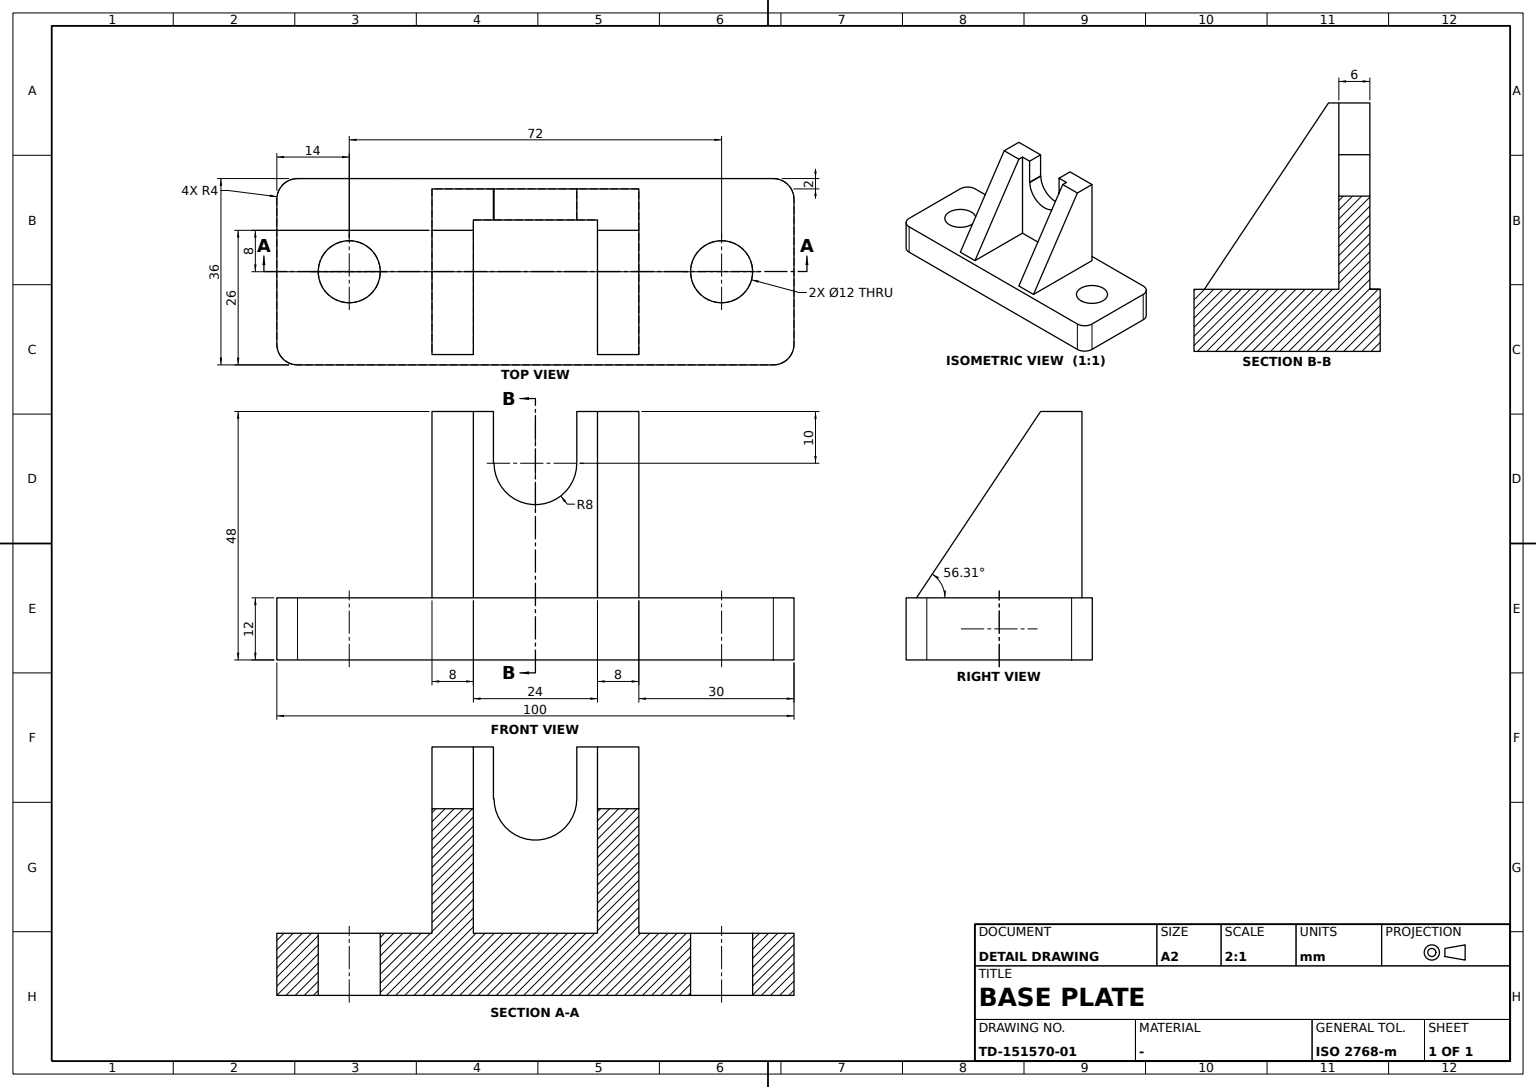
ISO-10303-21;
HEADER;
FILE_DESCRIPTION((''),'2;1');
FILE_NAME('','',(''),(''),'','','');
FILE_SCHEMA(('AUTOMOTIVE_DESIGN'));
ENDSEC;
DATA;
#1=APPLICATION_CONTEXT('');
#2=PRODUCT_CONTEXT('',#1,'mechanical');
#3=PRODUCT('','','',(#2));
#4=PRODUCT_DEFINITION_FORMATION('','',#3);
#5=PRODUCT_DEFINITION_CONTEXT('',#1,'design');
#6=PRODUCT_DEFINITION('','',#4,#5);
#7=PRODUCT_DEFINITION_SHAPE('','',#6);
#8=(LENGTH_UNIT()NAMED_UNIT(*)SI_UNIT(.MILLI.,.METRE.));
#9=(NAMED_UNIT(*)PLANE_ANGLE_UNIT()SI_UNIT($,.RADIAN.));
#10=(NAMED_UNIT(*)SI_UNIT($,.STERADIAN.)SOLID_ANGLE_UNIT());
#11=UNCERTAINTY_MEASURE_WITH_UNIT(LENGTH_MEASURE(0.005),#8,'distance_accuracy_value','');
#12=(GEOMETRIC_REPRESENTATION_CONTEXT(3)GLOBAL_UNCERTAINTY_ASSIGNED_CONTEXT((#11))GLOBAL_UNIT_ASSIGNED_CONTEXT((#8,#9,#10))REPRESENTATION_CONTEXT('',''));
#13=CARTESIAN_POINT('',(32.,100.,12.));
#14=VERTEX_POINT('',#13);
#15=CARTESIAN_POINT('',(4.,100.,12.));
#16=VERTEX_POINT('',#15);
#17=CARTESIAN_POINT('',(0.,100.,12.));
#18=DIRECTION('',(-1.,0.,0.));
#19=VECTOR('',#18,1000.);
#20=LINE('',#17,#19);
#21=EDGE_CURVE('',#14,#16,#20,.T.);
#22=ORIENTED_EDGE('',*,*,#21,.F.);
#23=CARTESIAN_POINT('',(32.,100.,0.));
#24=VERTEX_POINT('',#23);
#25=CARTESIAN_POINT('',(32.,100.,6.));
#26=DIRECTION('',(0.,0.,1.));
#27=VECTOR('',#26,1000.);
#28=LINE('',#25,#27);
#29=EDGE_CURVE('',#24,#14,#28,.T.);
#30=ORIENTED_EDGE('',*,*,#29,.F.);
#31=CARTESIAN_POINT('',(4.,100.,0.));
#32=VERTEX_POINT('',#31);
#33=CARTESIAN_POINT('',(0.,100.,0.));
#34=LINE('',#33,#19);
#35=EDGE_CURVE('',#24,#32,#34,.T.);
#36=ORIENTED_EDGE('',*,*,#35,.T.);
#37=CARTESIAN_POINT('',(4.,100.,6.));
#38=LINE('',#37,#27);
#39=EDGE_CURVE('',#32,#16,#38,.T.);
#40=ORIENTED_EDGE('',*,*,#39,.T.);
#41=EDGE_LOOP('',(#22,#30,#36,#40));
#42=FACE_BOUND('',#41,.T.);
#43=CARTESIAN_POINT('',(36.,100.,0.));
#44=DIRECTION('',(0.,1.,0.));
#45=AXIS2_PLACEMENT_3D('',#43,#44,#18);
#46=PLANE('',#45);
#47=ADVANCED_FACE('',(#42),#46,.T.);
#48=CARTESIAN_POINT('',(2.,70.,12.));
#49=VERTEX_POINT('',#48);
#50=CARTESIAN_POINT('',(2.,70.,48.));
#51=VERTEX_POINT('',#50);
#52=LINE('',#48,#27);
#53=EDGE_CURVE('',#49,#51,#52,.T.);
#54=ORIENTED_EDGE('',*,*,#53,.T.);
#55=CARTESIAN_POINT('',(10.,70.,48.));
#56=VERTEX_POINT('',#55);
#57=DIRECTION('',(1.,0.,0.));
#58=VECTOR('',#57,1000.);
#59=LINE('',#50,#58);
#60=EDGE_CURVE('',#51,#56,#59,.T.);
#61=ORIENTED_EDGE('',*,*,#60,.T.);
#62=CARTESIAN_POINT('',(34.,70.,12.));
#63=VERTEX_POINT('',#62);
#64=CARTESIAN_POINT('',(29.076923,70.,19.384615));
#65=DIRECTION('',(-0.554700196,0.,0.832050294));
#66=VECTOR('',#65,1000.);
#67=LINE('',#64,#66);
#68=EDGE_CURVE('',#63,#56,#67,.T.);
#69=ORIENTED_EDGE('',*,*,#68,.F.);
#70=CARTESIAN_POINT('',(0.,70.,12.));
#71=LINE('',#70,#19);
#72=EDGE_CURVE('',#63,#49,#71,.T.);
#73=ORIENTED_EDGE('',*,*,#72,.T.);
#74=EDGE_LOOP('',(#54,#61,#69,#73));
#75=FACE_BOUND('',#74,.T.);
#76=CARTESIAN_POINT('',(0.,70.,0.));
#77=AXIS2_PLACEMENT_3D('',#76,#44,#18);
#78=PLANE('',#77);
#79=ADVANCED_FACE('',(#75),#78,.T.);
#80=CARTESIAN_POINT('',(36.,96.,12.));
#81=VERTEX_POINT('',#80);
#82=CARTESIAN_POINT('',(32.,96.,12.));
#83=AXIS2_PLACEMENT_3D('',#82,#26,#57);
#84=CIRCLE('',#83,4.);
#85=EDGE_CURVE('',#81,#14,#84,.T.);
#86=ORIENTED_EDGE('',*,*,#85,.F.);
#87=CARTESIAN_POINT('',(36.,96.,0.));
#88=VERTEX_POINT('',#87);
#89=CARTESIAN_POINT('',(36.,96.,6.));
#90=LINE('',#89,#27);
#91=EDGE_CURVE('',#88,#81,#90,.T.);
#92=ORIENTED_EDGE('',*,*,#91,.F.);
#93=CARTESIAN_POINT('',(32.,96.,0.));
#94=AXIS2_PLACEMENT_3D('',#93,#26,#57);
#95=CIRCLE('',#94,4.);
#96=EDGE_CURVE('',#88,#24,#95,.T.);
#97=ORIENTED_EDGE('',*,*,#96,.T.);
#98=ORIENTED_EDGE('',*,*,#29,.T.);
#99=EDGE_LOOP('',(#86,#92,#97,#98));
#100=FACE_BOUND('',#99,.T.);
#101=CARTESIAN_POINT('',(32.,96.,6.));
#102=AXIS2_PLACEMENT_3D('',#101,#26,#44);
#103=CYLINDRICAL_SURFACE('',#102,4.);
#104=ADVANCED_FACE('',(#100),#103,.T.);
#105=CARTESIAN_POINT('',(0.,4.,12.));
#106=VERTEX_POINT('',#105);
#107=CARTESIAN_POINT('',(0.,96.,12.));
#108=VERTEX_POINT('',#107);
#109=CARTESIAN_POINT('',(0.,0.,12.));
#110=VECTOR('',#44,1000.);
#111=LINE('',#109,#110);
#112=EDGE_CURVE('',#106,#108,#111,.T.);
#113=ORIENTED_EDGE('',*,*,#112,.T.);
#114=CARTESIAN_POINT('',(0.,96.,0.));
#115=VERTEX_POINT('',#114);
#116=CARTESIAN_POINT('',(0.,96.,6.));
#117=LINE('',#116,#27);
#118=EDGE_CURVE('',#115,#108,#117,.T.);
#119=ORIENTED_EDGE('',*,*,#118,.F.);
#120=CARTESIAN_POINT('',(0.,4.,0.));
#121=VERTEX_POINT('',#120);
#122=CARTESIAN_POINT('',(0.,0.,0.));
#123=LINE('',#122,#110);
#124=EDGE_CURVE('',#121,#115,#123,.T.);
#125=ORIENTED_EDGE('',*,*,#124,.F.);
#126=CARTESIAN_POINT('',(0.,4.,6.));
#127=LINE('',#126,#27);
#128=EDGE_CURVE('',#121,#106,#127,.T.);
#129=ORIENTED_EDGE('',*,*,#128,.T.);
#130=EDGE_LOOP('',(#113,#119,#125,#129));
#131=FACE_BOUND('',#130,.T.);
#132=AXIS2_PLACEMENT_3D('',#122,#57,#44);
#133=PLANE('',#132);
#134=ADVANCED_FACE('',(#131),#133,.F.);
#135=CARTESIAN_POINT('',(2.,58.,48.));
#136=VERTEX_POINT('',#135);
#137=CARTESIAN_POINT('',(2.,58.,38.));
#138=VERTEX_POINT('',#137);
#139=CARTESIAN_POINT('',(2.,58.,12.));
#140=DIRECTION('',(0.,0.,-1.));
#141=VECTOR('',#140,1000.);
#142=LINE('',#139,#141);
#143=EDGE_CURVE('',#136,#138,#142,.T.);
#144=ORIENTED_EDGE('',*,*,#143,.T.);
#145=CARTESIAN_POINT('',(8.,58.,38.));
#146=VERTEX_POINT('',#145);
#147=CARTESIAN_POINT('',(19.66,58.,38.));
#148=LINE('',#147,#19);
#149=EDGE_CURVE('',#138,#146,#148,.F.);
#150=ORIENTED_EDGE('',*,*,#149,.T.);
#151=CARTESIAN_POINT('',(8.,58.,48.));
#152=VERTEX_POINT('',#151);
#153=CARTESIAN_POINT('',(8.,58.,48.236969));
#154=LINE('',#153,#27);
#155=EDGE_CURVE('',#146,#152,#154,.T.);
#156=ORIENTED_EDGE('',*,*,#155,.T.);
#157=LINE('',#135,#58);
#158=EDGE_CURVE('',#136,#152,#157,.T.);
#159=ORIENTED_EDGE('',*,*,#158,.F.);
#160=EDGE_LOOP('',(#144,#150,#156,#159));
#161=FACE_BOUND('',#160,.T.);
#162=CARTESIAN_POINT('',(2.,58.,48.236969));
#163=DIRECTION('',(0.,-1.,0.));
#164=AXIS2_PLACEMENT_3D('',#162,#163,#140);
#165=PLANE('',#164);
#166=ADVANCED_FACE('',(#161),#165,.T.);
#167=CARTESIAN_POINT('',(2.,41.879669,48.));
#168=VERTEX_POINT('',#167);
#169=CARTESIAN_POINT('',(8.,41.879669,48.));
#170=VERTEX_POINT('',#169);
#171=LINE('',#167,#58);
#172=EDGE_CURVE('',#168,#170,#171,.T.);
#173=ORIENTED_EDGE('',*,*,#172,.T.);
#174=CARTESIAN_POINT('',(8.,41.879669,38.));
#175=VERTEX_POINT('',#174);
#176=LINE('',#169,#27);
#177=EDGE_CURVE('',#175,#170,#176,.T.);
#178=ORIENTED_EDGE('',*,*,#177,.F.);
#179=CARTESIAN_POINT('',(2.,41.879669,38.));
#180=VERTEX_POINT('',#179);
#181=LINE('',#179,#58);
#182=EDGE_CURVE('',#180,#175,#181,.T.);
#183=ORIENTED_EDGE('',*,*,#182,.F.);
#184=CARTESIAN_POINT('',(2.,41.879669,12.));
#185=LINE('',#184,#27);
#186=EDGE_CURVE('',#180,#168,#185,.T.);
#187=ORIENTED_EDGE('',*,*,#186,.T.);
#188=EDGE_LOOP('',(#173,#178,#183,#187));
#189=FACE_BOUND('',#188,.T.);
#190=AXIS2_PLACEMENT_3D('',#179,#44,#26);
#191=PLANE('',#190);
#192=ADVANCED_FACE('',(#189),#191,.T.);
#193=CARTESIAN_POINT('',(8.,62.,48.));
#194=VERTEX_POINT('',#193);
#195=CARTESIAN_POINT('',(8.,62.,12.));
#196=VERTEX_POINT('',#195);
#197=LINE('',#193,#141);
#198=EDGE_CURVE('',#194,#196,#197,.T.);
#199=ORIENTED_EDGE('',*,*,#198,.T.);
#200=CARTESIAN_POINT('',(34.,62.,12.));
#201=VERTEX_POINT('',#200);
#202=LINE('',#195,#58);
#203=EDGE_CURVE('',#196,#201,#202,.T.);
#204=ORIENTED_EDGE('',*,*,#203,.T.);
#205=CARTESIAN_POINT('',(10.,62.,48.));
#206=VERTEX_POINT('',#205);
#207=CARTESIAN_POINT('',(9.384615,62.,48.923077));
#208=LINE('',#207,#66);
#209=EDGE_CURVE('',#201,#206,#208,.T.);
#210=ORIENTED_EDGE('',*,*,#209,.T.);
#211=CARTESIAN_POINT('',(2.,62.,48.));
#212=LINE('',#211,#58);
#213=EDGE_CURVE('',#194,#206,#212,.T.);
#214=ORIENTED_EDGE('',*,*,#213,.F.);
#215=EDGE_LOOP('',(#199,#204,#210,#214));
#216=FACE_BOUND('',#215,.T.);
#217=AXIS2_PLACEMENT_3D('',#193,#44,#57);
#218=PLANE('',#217);
#219=ADVANCED_FACE('',(#216),#218,.F.);
#220=ORIENTED_EDGE('',*,*,#68,.T.);
#221=CARTESIAN_POINT('',(10.,100.,48.));
#222=VECTOR('',#163,1000.);
#223=LINE('',#221,#222);
#224=EDGE_CURVE('',#56,#206,#223,.T.);
#225=ORIENTED_EDGE('',*,*,#224,.T.);
#226=ORIENTED_EDGE('',*,*,#209,.F.);
#227=CARTESIAN_POINT('',(34.,0.,12.));
#228=LINE('',#227,#222);
#229=EDGE_CURVE('',#63,#201,#228,.T.);
#230=ORIENTED_EDGE('',*,*,#229,.F.);
#231=EDGE_LOOP('',(#220,#225,#226,#230));
#232=FACE_BOUND('',#231,.T.);
#233=DIRECTION('',(-0.832050294,0.,-0.554700196));
#234=DIRECTION('',(0.554700196,0.,-0.832050294));
#235=AXIS2_PLACEMENT_3D('',#221,#233,#234);
#236=PLANE('',#235);
#237=ADVANCED_FACE('',(#232),#236,.F.);
#238=CARTESIAN_POINT('',(2.,42.,38.));
#239=VERTEX_POINT('',#238);
#240=CARTESIAN_POINT('',(2.,50.,38.));
#241=AXIS2_PLACEMENT_3D('',#240,#57,#140);
#242=CIRCLE('',#241,8.);
#243=EDGE_CURVE('',#138,#239,#242,.F.);
#244=ORIENTED_EDGE('',*,*,#243,.T.);
#245=CARTESIAN_POINT('',(8.,42.,38.));
#246=VERTEX_POINT('',#245);
#247=LINE('',#238,#19);
#248=EDGE_CURVE('',#239,#246,#247,.F.);
#249=ORIENTED_EDGE('',*,*,#248,.T.);
#250=CARTESIAN_POINT('',(8.,50.,38.));
#251=AXIS2_PLACEMENT_3D('',#250,#57,#140);
#252=CIRCLE('',#251,8.);
#253=EDGE_CURVE('',#246,#146,#252,.T.);
#254=ORIENTED_EDGE('',*,*,#253,.T.);
#255=ORIENTED_EDGE('',*,*,#149,.F.);
#256=EDGE_LOOP('',(#244,#249,#254,#255));
#257=FACE_BOUND('',#256,.T.);
#258=CARTESIAN_POINT('',(19.66,50.,38.));
#259=AXIS2_PLACEMENT_3D('',#258,#18,#163);
#260=CYLINDRICAL_SURFACE('',#259,8.);
#261=ADVANCED_FACE('',(#257),#260,.F.);
#262=CARTESIAN_POINT('',(36.,4.,0.));
#263=VERTEX_POINT('',#262);
#264=CARTESIAN_POINT('',(36.,4.,12.));
#265=VERTEX_POINT('',#264);
#266=CARTESIAN_POINT('',(36.,4.,6.));
#267=LINE('',#266,#27);
#268=EDGE_CURVE('',#263,#265,#267,.T.);
#269=ORIENTED_EDGE('',*,*,#268,.F.);
#270=CARTESIAN_POINT('',(36.,0.,0.));
#271=LINE('',#270,#222);
#272=EDGE_CURVE('',#88,#263,#271,.T.);
#273=ORIENTED_EDGE('',*,*,#272,.F.);
#274=ORIENTED_EDGE('',*,*,#91,.T.);
#275=CARTESIAN_POINT('',(36.,0.,12.));
#276=LINE('',#275,#222);
#277=EDGE_CURVE('',#81,#265,#276,.T.);
#278=ORIENTED_EDGE('',*,*,#277,.T.);
#279=EDGE_LOOP('',(#269,#273,#274,#278));
#280=FACE_BOUND('',#279,.T.);
#281=AXIS2_PLACEMENT_3D('',#43,#18,#163);
#282=PLANE('',#281);
#283=ADVANCED_FACE('',(#280),#282,.F.);
#284=ORIENTED_EDGE('',*,*,#253,.F.);
#285=CARTESIAN_POINT('',(8.,62.,38.));
#286=LINE('',#285,#222);
#287=EDGE_CURVE('',#246,#175,#286,.T.);
#288=ORIENTED_EDGE('',*,*,#287,.T.);
#289=ORIENTED_EDGE('',*,*,#177,.T.);
#290=CARTESIAN_POINT('',(8.,38.,48.));
#291=VERTEX_POINT('',#290);
#292=CARTESIAN_POINT('',(8.,100.,48.));
#293=LINE('',#292,#222);
#294=EDGE_CURVE('',#170,#291,#293,.T.);
#295=ORIENTED_EDGE('',*,*,#294,.T.);
#296=CARTESIAN_POINT('',(8.,38.,12.));
#297=VERTEX_POINT('',#296);
#298=LINE('',#290,#141);
#299=EDGE_CURVE('',#291,#297,#298,.T.);
#300=ORIENTED_EDGE('',*,*,#299,.T.);
#301=LINE('',#195,#222);
#302=EDGE_CURVE('',#196,#297,#301,.T.);
#303=ORIENTED_EDGE('',*,*,#302,.F.);
#304=ORIENTED_EDGE('',*,*,#198,.F.);
#305=EDGE_CURVE('',#194,#152,#293,.T.);
#306=ORIENTED_EDGE('',*,*,#305,.T.);
#307=ORIENTED_EDGE('',*,*,#155,.F.);
#308=EDGE_LOOP('',(#284,#288,#289,#295,#300,#303,#304,#306,#307));
#309=FACE_BOUND('',#308,.T.);
#310=AXIS2_PLACEMENT_3D('',#193,#57,#163);
#311=PLANE('',#310);
#312=ADVANCED_FACE('',(#309),#311,.T.);
#313=CARTESIAN_POINT('',(34.,38.,12.));
#314=VERTEX_POINT('',#313);
#315=CARTESIAN_POINT('',(10.,38.,48.));
#316=VERTEX_POINT('',#315);
#317=LINE('',#315,#66);
#318=EDGE_CURVE('',#314,#316,#317,.T.);
#319=ORIENTED_EDGE('',*,*,#318,.F.);
#320=LINE('',#313,#19);
#321=EDGE_CURVE('',#314,#297,#320,.T.);
#322=ORIENTED_EDGE('',*,*,#321,.T.);
#323=ORIENTED_EDGE('',*,*,#299,.F.);
#324=CARTESIAN_POINT('',(2.,38.,48.));
#325=LINE('',#324,#19);
#326=EDGE_CURVE('',#316,#291,#325,.T.);
#327=ORIENTED_EDGE('',*,*,#326,.F.);
#328=EDGE_LOOP('',(#319,#322,#323,#327));
#329=FACE_BOUND('',#328,.T.);
#330=CARTESIAN_POINT('',(34.,38.,48.));
#331=AXIS2_PLACEMENT_3D('',#330,#163,#18);
#332=PLANE('',#331);
#333=ADVANCED_FACE('',(#329),#332,.F.);
#334=CARTESIAN_POINT('',(2.,30.,48.));
#335=VERTEX_POINT('',#334);
#336=CARTESIAN_POINT('',(10.,30.,48.));
#337=VERTEX_POINT('',#336);
#338=LINE('',#334,#58);
#339=EDGE_CURVE('',#335,#337,#338,.T.);
#340=ORIENTED_EDGE('',*,*,#339,.T.);
#341=EDGE_CURVE('',#316,#337,#223,.T.);
#342=ORIENTED_EDGE('',*,*,#341,.F.);
#343=ORIENTED_EDGE('',*,*,#326,.T.);
#344=ORIENTED_EDGE('',*,*,#294,.F.);
#345=ORIENTED_EDGE('',*,*,#172,.F.);
#346=CARTESIAN_POINT('',(2.,100.,48.));
#347=LINE('',#346,#222);
#348=EDGE_CURVE('',#168,#335,#347,.T.);
#349=ORIENTED_EDGE('',*,*,#348,.T.);
#350=EDGE_LOOP('',(#340,#342,#343,#344,#345,#349));
#351=FACE_BOUND('',#350,.T.);
#352=AXIS2_PLACEMENT_3D('',#346,#140,#57);
#353=PLANE('',#352);
#354=ADVANCED_FACE('',(#351),#353,.F.);
#355=CARTESIAN_POINT('',(24.,86.,12.));
#356=VERTEX_POINT('',#355);
#357=CARTESIAN_POINT('',(18.,86.,12.));
#358=AXIS2_PLACEMENT_3D('',#357,#26,#57);
#359=CIRCLE('',#358,6.);
#360=EDGE_CURVE('',#356,#356,#359,.T.);
#361=ORIENTED_EDGE('',*,*,#360,.F.);
#362=EDGE_LOOP('',(#361));
#363=FACE_BOUND('',#362,.T.);
#364=ORIENTED_EDGE('',*,*,#112,.F.);
#365=CARTESIAN_POINT('',(4.,0.,12.));
#366=VERTEX_POINT('',#365);
#367=CARTESIAN_POINT('',(4.,4.,12.));
#368=AXIS2_PLACEMENT_3D('',#367,#26,#57);
#369=CIRCLE('',#368,4.);
#370=EDGE_CURVE('',#106,#366,#369,.T.);
#371=ORIENTED_EDGE('',*,*,#370,.T.);
#372=CARTESIAN_POINT('',(32.,0.,12.));
#373=VERTEX_POINT('',#372);
#374=LINE('',#109,#58);
#375=EDGE_CURVE('',#366,#373,#374,.T.);
#376=ORIENTED_EDGE('',*,*,#375,.T.);
#377=CARTESIAN_POINT('',(32.,4.,12.));
#378=AXIS2_PLACEMENT_3D('',#377,#26,#57);
#379=CIRCLE('',#378,4.);
#380=EDGE_CURVE('',#373,#265,#379,.T.);
#381=ORIENTED_EDGE('',*,*,#380,.T.);
#382=ORIENTED_EDGE('',*,*,#277,.F.);
#383=ORIENTED_EDGE('',*,*,#85,.T.);
#384=ORIENTED_EDGE('',*,*,#21,.T.);
#385=CARTESIAN_POINT('',(4.,96.,12.));
#386=AXIS2_PLACEMENT_3D('',#385,#26,#57);
#387=CIRCLE('',#386,4.);
#388=EDGE_CURVE('',#16,#108,#387,.T.);
#389=ORIENTED_EDGE('',*,*,#388,.T.);
#390=EDGE_LOOP('',(#364,#371,#376,#381,#382,#383,#384,#389));
#391=FACE_BOUND('',#390,.T.);
#392=CARTESIAN_POINT('',(24.,14.,12.));
#393=VERTEX_POINT('',#392);
#394=CARTESIAN_POINT('',(18.,14.,12.));
#395=AXIS2_PLACEMENT_3D('',#394,#26,#57);
#396=CIRCLE('',#395,6.);
#397=EDGE_CURVE('',#393,#393,#396,.T.);
#398=ORIENTED_EDGE('',*,*,#397,.F.);
#399=EDGE_LOOP('',(#398));
#400=FACE_BOUND('',#399,.T.);
#401=ORIENTED_EDGE('',*,*,#203,.F.);
#402=ORIENTED_EDGE('',*,*,#302,.T.);
#403=ORIENTED_EDGE('',*,*,#321,.F.);
#404=CARTESIAN_POINT('',(34.,30.,12.));
#405=VERTEX_POINT('',#404);
#406=EDGE_CURVE('',#314,#405,#228,.T.);
#407=ORIENTED_EDGE('',*,*,#406,.T.);
#408=CARTESIAN_POINT('',(2.,30.,12.));
#409=VERTEX_POINT('',#408);
#410=LINE('',#408,#58);
#411=EDGE_CURVE('',#409,#405,#410,.T.);
#412=ORIENTED_EDGE('',*,*,#411,.F.);
#413=CARTESIAN_POINT('',(2.,100.,12.));
#414=LINE('',#413,#222);
#415=EDGE_CURVE('',#49,#409,#414,.T.);
#416=ORIENTED_EDGE('',*,*,#415,.F.);
#417=ORIENTED_EDGE('',*,*,#72,.F.);
#418=ORIENTED_EDGE('',*,*,#229,.T.);
#419=EDGE_LOOP('',(#401,#402,#403,#407,#412,#416,#417,#418));
#420=FACE_BOUND('',#419,.T.);
#421=AXIS2_PLACEMENT_3D('',#109,#26,#44);
#422=PLANE('',#421);
#423=ADVANCED_FACE('',(#363,#391,#400,#420),#422,.T.);
#424=CARTESIAN_POINT('',(2.,100.,38.));
#425=LINE('',#424,#222);
#426=EDGE_CURVE('',#239,#180,#425,.T.);
#427=ORIENTED_EDGE('',*,*,#426,.T.);
#428=ORIENTED_EDGE('',*,*,#182,.T.);
#429=ORIENTED_EDGE('',*,*,#287,.F.);
#430=ORIENTED_EDGE('',*,*,#248,.F.);
#431=EDGE_LOOP('',(#427,#428,#429,#430));
#432=FACE_BOUND('',#431,.T.);
#433=AXIS2_PLACEMENT_3D('',#238,#26,#163);
#434=PLANE('',#433);
#435=ADVANCED_FACE('',(#432),#434,.T.);
#436=CARTESIAN_POINT('',(32.,0.,0.));
#437=VERTEX_POINT('',#436);
#438=CARTESIAN_POINT('',(32.,0.,6.));
#439=LINE('',#438,#27);
#440=EDGE_CURVE('',#437,#373,#439,.T.);
#441=ORIENTED_EDGE('',*,*,#440,.F.);
#442=CARTESIAN_POINT('',(32.,4.,0.));
#443=AXIS2_PLACEMENT_3D('',#442,#26,#57);
#444=CIRCLE('',#443,4.);
#445=EDGE_CURVE('',#437,#263,#444,.T.);
#446=ORIENTED_EDGE('',*,*,#445,.T.);
#447=ORIENTED_EDGE('',*,*,#268,.T.);
#448=ORIENTED_EDGE('',*,*,#380,.F.);
#449=EDGE_LOOP('',(#441,#446,#447,#448));
#450=FACE_BOUND('',#449,.T.);
#451=CARTESIAN_POINT('',(32.,4.,6.));
#452=AXIS2_PLACEMENT_3D('',#451,#26,#57);
#453=CYLINDRICAL_SURFACE('',#452,4.);
#454=ADVANCED_FACE('',(#450),#453,.T.);
#455=ORIENTED_EDGE('',*,*,#411,.T.);
#456=VECTOR('',#234,1000.);
#457=LINE('',#336,#456);
#458=EDGE_CURVE('',#337,#405,#457,.T.);
#459=ORIENTED_EDGE('',*,*,#458,.F.);
#460=ORIENTED_EDGE('',*,*,#339,.F.);
#461=LINE('',#408,#27);
#462=EDGE_CURVE('',#409,#335,#461,.T.);
#463=ORIENTED_EDGE('',*,*,#462,.F.);
#464=EDGE_LOOP('',(#455,#459,#460,#463));
#465=FACE_BOUND('',#464,.T.);
#466=AXIS2_PLACEMENT_3D('',#408,#44,#26);
#467=PLANE('',#466);
#468=ADVANCED_FACE('',(#465),#467,.F.);
#469=ORIENTED_EDGE('',*,*,#158,.T.);
#470=ORIENTED_EDGE('',*,*,#305,.F.);
#471=ORIENTED_EDGE('',*,*,#213,.T.);
#472=ORIENTED_EDGE('',*,*,#224,.F.);
#473=ORIENTED_EDGE('',*,*,#60,.F.);
#474=EDGE_CURVE('',#51,#136,#347,.T.);
#475=ORIENTED_EDGE('',*,*,#474,.T.);
#476=EDGE_LOOP('',(#469,#470,#471,#472,#473,#475));
#477=FACE_BOUND('',#476,.T.);
#478=ADVANCED_FACE('',(#477),#353,.F.);
#479=ORIENTED_EDGE('',*,*,#440,.T.);
#480=ORIENTED_EDGE('',*,*,#375,.F.);
#481=CARTESIAN_POINT('',(4.,0.,0.));
#482=VERTEX_POINT('',#481);
#483=CARTESIAN_POINT('',(4.,0.,6.));
#484=LINE('',#483,#27);
#485=EDGE_CURVE('',#482,#366,#484,.T.);
#486=ORIENTED_EDGE('',*,*,#485,.F.);
#487=LINE('',#122,#58);
#488=EDGE_CURVE('',#482,#437,#487,.T.);
#489=ORIENTED_EDGE('',*,*,#488,.T.);
#490=EDGE_LOOP('',(#479,#480,#486,#489));
#491=FACE_BOUND('',#490,.T.);
#492=AXIS2_PLACEMENT_3D('',#122,#163,#57);
#493=PLANE('',#492);
#494=ADVANCED_FACE('',(#491),#493,.T.);
#495=CARTESIAN_POINT('',(24.,86.,0.));
#496=VERTEX_POINT('',#495);
#497=CARTESIAN_POINT('',(18.,86.,0.));
#498=AXIS2_PLACEMENT_3D('',#497,#26,#57);
#499=CIRCLE('',#498,6.);
#500=EDGE_CURVE('',#496,#496,#499,.T.);
#501=ORIENTED_EDGE('',*,*,#500,.F.);
#502=EDGE_LOOP('',(#501));
#503=FACE_BOUND('',#502,.T.);
#504=ORIENTED_EDGE('',*,*,#360,.T.);
#505=EDGE_LOOP('',(#504));
#506=FACE_BOUND('',#505,.T.);
#507=CARTESIAN_POINT('',(18.,86.,5.34));
#508=AXIS2_PLACEMENT_3D('',#507,#26,#57);
#509=CYLINDRICAL_SURFACE('',#508,6.);
#510=ADVANCED_FACE('',(#503,#506),#509,.F.);
#511=ORIENTED_EDGE('',*,*,#406,.F.);
#512=ORIENTED_EDGE('',*,*,#318,.T.);
#513=ORIENTED_EDGE('',*,*,#341,.T.);
#514=ORIENTED_EDGE('',*,*,#458,.T.);
#515=EDGE_LOOP('',(#511,#512,#513,#514));
#516=FACE_BOUND('',#515,.T.);
#517=ADVANCED_FACE('',(#516),#236,.F.);
#518=CARTESIAN_POINT('',(4.,4.,0.));
#519=AXIS2_PLACEMENT_3D('',#518,#26,#57);
#520=CIRCLE('',#519,4.);
#521=EDGE_CURVE('',#121,#482,#520,.T.);
#522=ORIENTED_EDGE('',*,*,#521,.F.);
#523=ORIENTED_EDGE('',*,*,#124,.T.);
#524=CARTESIAN_POINT('',(4.,96.,0.));
#525=AXIS2_PLACEMENT_3D('',#524,#26,#57);
#526=CIRCLE('',#525,4.);
#527=EDGE_CURVE('',#32,#115,#526,.T.);
#528=ORIENTED_EDGE('',*,*,#527,.F.);
#529=ORIENTED_EDGE('',*,*,#35,.F.);
#530=ORIENTED_EDGE('',*,*,#96,.F.);
#531=ORIENTED_EDGE('',*,*,#272,.T.);
#532=ORIENTED_EDGE('',*,*,#445,.F.);
#533=ORIENTED_EDGE('',*,*,#488,.F.);
#534=EDGE_LOOP('',(#522,#523,#528,#529,#530,#531,#532,#533));
#535=FACE_BOUND('',#534,.T.);
#536=CARTESIAN_POINT('',(24.,14.,0.));
#537=VERTEX_POINT('',#536);
#538=CARTESIAN_POINT('',(18.,14.,0.));
#539=AXIS2_PLACEMENT_3D('',#538,#26,#57);
#540=CIRCLE('',#539,6.);
#541=EDGE_CURVE('',#537,#537,#540,.T.);
#542=ORIENTED_EDGE('',*,*,#541,.T.);
#543=EDGE_LOOP('',(#542));
#544=FACE_BOUND('',#543,.T.);
#545=ORIENTED_EDGE('',*,*,#500,.T.);
#546=EDGE_LOOP('',(#545));
#547=FACE_BOUND('',#546,.T.);
#548=AXIS2_PLACEMENT_3D('',#122,#26,#44);
#549=PLANE('',#548);
#550=ADVANCED_FACE('',(#535,#544,#547),#549,.F.);
#551=ORIENTED_EDGE('',*,*,#474,.F.);
#552=ORIENTED_EDGE('',*,*,#53,.F.);
#553=ORIENTED_EDGE('',*,*,#415,.T.);
#554=ORIENTED_EDGE('',*,*,#462,.T.);
#555=ORIENTED_EDGE('',*,*,#348,.F.);
#556=ORIENTED_EDGE('',*,*,#186,.F.);
#557=ORIENTED_EDGE('',*,*,#426,.F.);
#558=ORIENTED_EDGE('',*,*,#243,.F.);
#559=ORIENTED_EDGE('',*,*,#143,.F.);
#560=EDGE_LOOP('',(#551,#552,#553,#554,#555,#556,#557,#558,#559));
#561=FACE_BOUND('',#560,.T.);
#562=AXIS2_PLACEMENT_3D('',#413,#57,#26);
#563=PLANE('',#562);
#564=ADVANCED_FACE('',(#561),#563,.F.);
#565=ORIENTED_EDGE('',*,*,#397,.T.);
#566=EDGE_LOOP('',(#565));
#567=FACE_BOUND('',#566,.T.);
#568=ORIENTED_EDGE('',*,*,#541,.F.);
#569=EDGE_LOOP('',(#568));
#570=FACE_BOUND('',#569,.T.);
#571=CARTESIAN_POINT('',(18.,14.,5.34));
#572=AXIS2_PLACEMENT_3D('',#571,#26,#57);
#573=CYLINDRICAL_SURFACE('',#572,6.);
#574=ADVANCED_FACE('',(#567,#570),#573,.F.);
#575=ORIENTED_EDGE('',*,*,#128,.F.);
#576=ORIENTED_EDGE('',*,*,#521,.T.);
#577=ORIENTED_EDGE('',*,*,#485,.T.);
#578=ORIENTED_EDGE('',*,*,#370,.F.);
#579=EDGE_LOOP('',(#575,#576,#577,#578));
#580=FACE_BOUND('',#579,.T.);
#581=CARTESIAN_POINT('',(4.,4.,6.));
#582=AXIS2_PLACEMENT_3D('',#581,#26,#163);
#583=CYLINDRICAL_SURFACE('',#582,4.);
#584=ADVANCED_FACE('',(#580),#583,.T.);
#585=ORIENTED_EDGE('',*,*,#39,.F.);
#586=ORIENTED_EDGE('',*,*,#527,.T.);
#587=ORIENTED_EDGE('',*,*,#118,.T.);
#588=ORIENTED_EDGE('',*,*,#388,.F.);
#589=EDGE_LOOP('',(#585,#586,#587,#588));
#590=FACE_BOUND('',#589,.T.);
#591=CARTESIAN_POINT('',(4.,96.,6.));
#592=AXIS2_PLACEMENT_3D('',#591,#26,#18);
#593=CYLINDRICAL_SURFACE('',#592,4.);
#594=ADVANCED_FACE('',(#590),#593,.T.);
#595=CLOSED_SHELL('',(#47,#79,#104,#134,#166,#192,#219,#237,#261,#283,#312,#333,#354,#423,#435,#454,#468,#478,#494,#510,#517,#550,#564,#574,#584,#594));
#596=MANIFOLD_SOLID_BREP('',#595);
#597=ADVANCED_BREP_SHAPE_REPRESENTATION('',(#596),#12);
#598=SHAPE_DEFINITION_REPRESENTATION(#7,#597);
ENDSEC;
END-ISO-10303-21;
